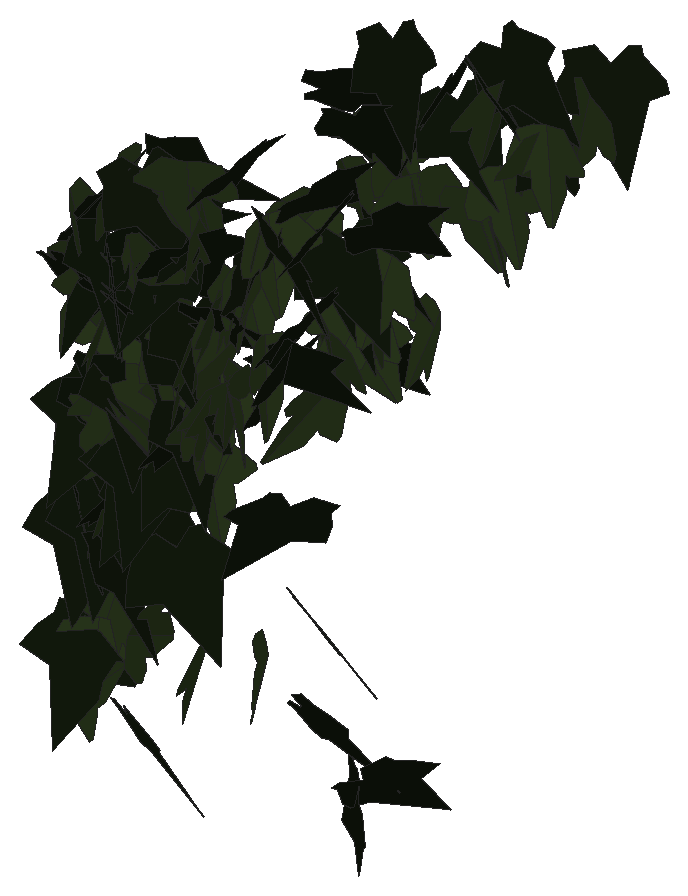
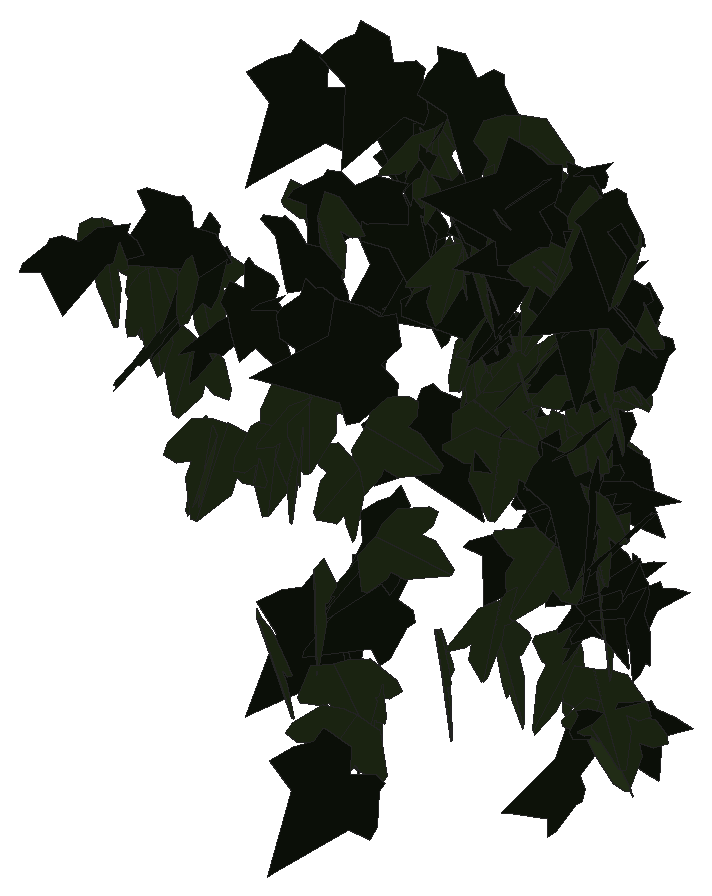
# SketchUp Ruby script. Lengths in inches.
U = 1.inch
M = Sketchup.active_model
def pt(a) = Geom::Point3d.new(a.map { |v| v * U })
def face(e, loops, mat)
  f = e.add_face(loops[0].map { |a| pt(a) })
  loops[1..].each { |l| e.add_face(l.map { |a| pt(a) }).erase! }
  f.material = f.back_material = mat if mat
  f
end
# faces: each face lists its corners as indices into pts; further lists are holes
def faces(e, pts, list, mat = nil) = list.each { |f| face(e, (f[0].is_a?(Array) ? f : [f]).map { |l| l.map { |i| pts[i] } }, mat) }
# xy, xz, yz: faces in a plane at the given z, y or x. An outline is a flat list of corners, or four numbers for a rectangle; further outlines are holes
def ring(l) = l.size == 4 ? [[l[0], l[1]], [l[2], l[1]], [l[2], l[3]], [l[0], l[3]]] : l.each_slice(2).to_a
def flat(e, list, mat, &to3) = list.each { |f| face(e, (f[0].is_a?(Array) ? f : [f]).map { |l| ring(l).map { |u, v| to3.(u, v) } }, mat) }
def xy(e, z, list, mat = nil) = flat(e, list, mat) { |x, y| [x, y, z] }
def xz(e, y, list, mat = nil) = flat(e, list, mat) { |x, z| [x, y, z] }
def yz(e, x, list, mat = nil) = flat(e, list, mat) { |y, z| [x, y, z] }
def lines(e, pts, list) = list.each { |a, b| e.add_line(pt(pts[a]), pt(pts[b])) }
# prism: a flat outline (further loops are holes) pulled along v
def prism(e, loops, v, mat = nil)
  f = face(e, loops, mat); d = Geom::Vector3d.new(v.map { |x| x * U })
  f.pushpull(f.normal.samedirection?(d) ? d.length : -d.length)
end
def box(e, o, s, mat = nil) = prism(e, [[o, [o[0] + s[0], o[1], o[2]], [o[0] + s[0], o[1] + s[1], o[2]], [o[0], o[1] + s[1], o[2]]]], [0, 0, s[2]], mat)
def at(x, y, z, deg = 0) = Geom::Transformation.translation(pt([x, y, z])) * Geom::Transformation.rotation(ORIGIN, Z_AXIS, deg.degrees)
def axes(o, x, y, z) = Geom::Transformation.new([*x, 0, *y, 0, *z, 0, *pt(o).to_a, 1])
def part(name) = M.definitions.add(name)
# library, detail: a bought-in or finely detailed component or shape, given as its bounding box
def library(name, o, s) = part(name).tap { |d| box(d.entities, o, s) }
def detail(e, o, s) = box(e.add_group.entities, o, s)
def put(e, d, t, mat = nil) = e.add_instance(d, t).tap { |i| i.material = mat if mat }
def group(e, t, mat = nil) = e.add_group.tap { |g| g.transformation = t; g.material = mat if mat }.entities
root = M.entities
M.materials.add("efeu1").color = [18, 25, 13]
M.materials.add("efeu2").color = [43, 57, 29]
c1 = part("ivyleaf_9")
p = [[1.54,2.16,1.25],[1.36,2.04,1.19],[-0.21,0.99,0.68],[-0.71,1.11,0.82],[-0.85,0.86,0.67],[-0.8,0.17,0.21],
  [-0.9,-0.01,0.1],[-0.67,-0.16,-0.02],[-0.08,-0.08,-0.05],[-0.03,-0.6,-0.4],[0.65,-0.88,-0.66],[0.83,-0.6,-0.49],
  [1.29,-0.42,-0.43],[1.8125,-0.07,-0.26],[1.21,0.44,0.15]]
faces(c1.entities,p,[[0,1,2,3,4,5,6,7,8,9,10,11,12,13,14]],"efeu1")
c2 = part("ivyleaf_10")
p = [[0,0.5,-0.03],[-0.0625,2.02,-0.43],[-0.19,2.01,-0.46],[-0.54,1.05,-0.29],[-0.52,0.625,-0.18],[-0.83,0.76,-0.28],
  [-1.16,0.64,-0.33],[-1.15,0.33,-0.24],[-0.77,-0.39,0.02],[-0.3,-0.51,0.16],[0.04,-0.48,0.23],[-0.02,2.01,-0.4375],
  [-0.06,2.01,-0.43],[0.04,-0.49,0.23],[0.67,-0.49,0.14],[1.38,0.36,-0.2],[1.375,0.51,-0.24],[0.81,0.65,-0.19],
  [0.62,0.59,-0.15],[0.6,1.09,-0.28],[0.5,1.23,-0.31]]
faces(c2.entities,p,[[0,1,2,3,4,5,6,7,8,9,10],[11,12,0,13,14,15,16,17,18,19,20]],"efeu2")
put(root,c1,axes([47.6,222.98,241.15],[0.28604,-0.36805,0.18089],[0.10443,-0.14791,-0.46607],[0.39658,0.30441,-0.00775]))
put(root,c2,axes([47.37,222.98,241.04],[-0.14695,0.39138,-0.27427],[-0.05131,-0.2982,-0.39805],[-0.47515,-0.08884,0.12781]))
put(root,c1,axes([45.58,223.13,237.33],[-0.35883,-0.34791,-0.01403],[0.06783,-0.05009,-0.49284],[0.34152,-0.3556,0.08314]))
put(root,c1,axes([45.51,223.15,237.27],[-0.12119,-0.47664,0.09015],[-0.0015,-0.09255,-0.49136],[0.48509,-0.11937,0.021]))
put(root,c1,axes([45.03,222.95,235.92],[0.29145,-0.40527,0.02852],[0.01419,-0.02492,-0.49918],[0.40602,0.29178,-0.00302]))
put(root,c1,axes([44.71,223.06,234.62],[-0.35713,-0.33851,-0.08871],[0.0584,0.06733,-0.49199],[0.34503,-0.36177,-0.00856]))
put(root,c2,axes([45.1875,222.87,237.78],[-0.41971,-0.04897,0.26729],[-0.25366,-0.10581,-0.41769],[0.09747,-0.48622,0.06398]))
put(root,c2,axes([46.34,222.83,241.66],[-0.44608,-0.22491,0.02083],[-0.01528,-0.01595,-0.49951],[0.22535,-0.44628,0.00736]))
put(root,c1,axes([44.92,223.09,240.11],[0.07095,-0.49203,0.05358],[0.00626,-0.05323,-0.49712],[0.4949,0.07121,-0.0014]))
put(root,c1,axes([44.87,223.05,240.09],[-0.42662,-0.06259,-0.25313],[0.25792,-0.02984,-0.4273],[0.03838,-0.49517,0.05775]))
put(root,c2,axes([47.5,222.91,239.53],[-0.0551,0.4761,-0.14244],[-0.00281,-0.14361,-0.47892],[-0.49695,-0.05198,0.0185]))
put(root,c2,axes([44.7,223.02,233.87],[0.14859,-0.36574,-0.30685],[0.26499,-0.20414,0.37163],[-0.39712,-0.27306,0.13317]))
put(root,c1,axes([46.1,222.92,236.33],[-0.11764,-0.34267,-0.34459],[0.22985,0.27315,-0.35009],[0.42817,-0.24077,0.09326]))
put(root,c2,axes([46.55,223.02,239.73],[0.24723,-0.41637,0.12454],[0.07019,-0.10314,-0.48418],[0.42889,0.25689,0.00745]))
put(root,c2,axes([44.64,222.82,240.6],[-0.20643,0.45476,-0.02403],[-0.00018,-0.02646,-0.4993],[-0.4554,-0.20613,0.01108]))
put(root,c2,axes([45.82,222.85,240.27],[-0.46736,0.00036,0.1777],[-0.17738,-0.03109,-0.46644],[0.01072,-0.49903,0.02919]))
put(root,c1,axes([47.76,222.95,237.49],[-0.01009,0.32824,-0.37704],[-0.10454,-0.37016,-0.31946],[-0.48885,0.07239,0.0761]))
put(root,c1,axes([45.58,222.93,241.36],[0.08904,-0.4323,-0.23493],[0.06047,0.24655,-0.43076],[0.48828,0.04829,0.09619]))
put(root,c1,axes([45.23,222.63,241.15],[-0.06272,0.47356,0.14768],[-0.06747,0.13933,-0.47543],[-0.49144,-0.07957,0.04643]))
put(root,c1,axes([44.9,223.15,239.875],[0.03196,-0.00013,-0.49898],[0.47505,-0.15296,0.03047],[-0.15266,-0.47603,-0.00966]))
put(root,c2,axes([46.62,223.02,238.57],[0.13599,-0.47813,0.05381],[0.01,-0.0531,-0.49707],[0.48105,0.13627,-0.00488]))
put(root,c2,axes([46.13,223.06,239.05],[0.2724,-0.40437,0.11081],[0.07632,-0.08211,-0.48727],[0.41228,0.28238,0.01699]))
put(root,c2,axes([46.47,223.03,238.36],[0.03089,-0.49446,0.0675],[0.00051,-0.06759,-0.49541],[0.49904,0.03067,-0.00368]))
put(root,c1,axes([45.93,223.17,240.29],[-0.45951,-0.0891,-0.17581],[0.1917,-0.09836,-0.4512],[0.04582,-0.48207,0.12455]))
put(root,c2,axes([46.26,222.93,241.26],[-0.41596,-0.09564,0.26044],[-0.25167,-0.06753,-0.42674],[0.1168,-0.4861,0.00804]))
put(root,c2,axes([44.64,223.17,239.54],[-0.00824,-0.42593,0.26176],[0.03234,-0.2617,-0.42481],[0.49888,0.00993,0.03186]))
put(root,c2,axes([45.09,222.99,238.12],[-0.0935,0.04522,-0.48909],[0.46125,-0.16305,-0.10325],[-0.16883,-0.4705,-0.01123]))
put(root,c1,axes([47.1,222.65,242.05],[0.00869,0.49275,0.08441],[-0.03311,0.0848,-0.49164],[-0.49883,0.00295,0.0341]))
put(root,c2,axes([47.56,222.9,241.22],[0.10794,0.48798,-0.01486],[0.00353,-0.01599,-0.49973],[-0.4882,0.10778,-0.00689]))
put(root,c2,axes([44.77,222.91,239.87],[-0.49251,-0.02626,0.08211],[-0.08067,-0.02749,-0.49268],[0.03039,-0.49855,0.02284]))
put(root,c1,axes([46.09,223.15,238.11],[0.11345,-0.48539,0.0391],[0.01037,-0.03773,-0.49847],[0.48685,0.11391,0.0015]))
put(root,c1,axes([48.16,222.86,234.87],[0.48306,-0.09603,0.08621],[0.08554,-0.0118,-0.49249],[0.09662,0.49055,0.00503]))
put(root,c1,axes([48.375,222.78,241.625],[-0.16599,0.4716,0.00615],[0.00009,0.00655,-0.49996],[-0.47164,-0.16597,-0.00226]))
put(root,c2,axes([44.9,222.98,239.15],[0.21957,-0.44175,-0.08151],[-0.04878,0.06675,-0.49312],[0.44656,0.2245,-0.01379]))
put(root,c1,axes([47.67,222.55,239.13],[0.09531,0.21275,0.44233],[0.10934,0.43006,-0.23041],[-0.4785,0.14065,0.03545]))
put(root,c2,axes([46.34,223.05,234.98],[0.20444,-0.45618,0.0102],[0.00335,-0.00967,-0.4999],[0.45628,0.20447,-0.0009]))
put(root,c1,axes([47.47,222.68,240.75],[-0.13862,0.38287,0.29017],[-0.12009,0.2648,-0.40677],[-0.46515,-0.18247,0.01855]))
put(root,c1,axes([44.87,222.89,239.39],[0.46589,-0.1151,0.14037],[0.13818,-0.02586,-0.47983],[0.11771,0.48588,0.00772]))
put(root,c1,axes([44.74,223.25,236.36],[-0.05848,-0.49573,0.02878],[-0.0111,-0.02767,-0.49911],[0.49644,-0.05902,-0.00777]))
put(root,c1,axes([44.375,222.84,239.73],[0.49918,-0.02713,0.00929],[0.01052,0.02252,-0.49938],[0.02668,0.49876,0.02305]))
put(root,c1,axes([44.5,223.24,236.21],[-0.14334,-0.47866,-0.01836],[0.02143,0.01274,-0.49938],[0.47853,-0.14395,0.01687]))
put(root,c1,axes([48.03,222.84,240.19],[-0.12703,0.48156,-0.04433],[-0.00004,-0.04584,-0.49789],[-0.48359,-0.12649,0.01168]))
put(root,c2,axes([46.77,222.99,238.75],[-0.08312,-0.48753,-0.07349],[-0.0059,0.0755,-0.49423],[0.49301,-0.0813,-0.01831]))
put(root,c2,axes([47.1,223.01,240.28],[0.31561,-0.3772,-0.09003],[-0.0171,0.10244,-0.4891],[0.38742,0.31181,0.05176]))
put(root,c1,axes([44.18,223.2,236.24],[0.06907,-0.03833,-0.49372],[0.49411,-0.02782,0.07128],[-0.03293,-0.49775,0.03404]))
put(root,c2,axes([44.71,223.04,234.6],[0.46843,0.17468,-0.00779],[-0.01618,0.02112,-0.49929],[-0.17411,0.46802,0.02544]))
put(root,c1,axes([44.68,223.31,237.74],[-0.39387,-0.30628,-0.03253],[0.06808,-0.03508,-0.4941],[0.30038,-0.39365,0.06933]))
put(root,c1,axes([46.29,222.79,240.62],[0.21685,0.44719,-0.05476],[-0.0266,-0.04796,-0.49698],[-0.44975,0.21845,0.00299]))
put(root,c1,axes([46.1,223.1875,239.46],[0.09539,-0.48653,-0.06474],[-0.02045,0.06195,-0.49573],[0.49039,0.09722,-0.00808]))
put(root,c1,axes([45.26,223.08,233.65],[0.39625,-0.2893,0.09641],[0.07937,-0.05479,-0.49061],[0.29443,0.40411,0.0025]))
put(root,c1,axes([44.68,222.9375,238.1875],[0.10643,0.0448,-0.48648],[0.3771,0.30901,0.11095],[0.3106,-0.39052,0.03198]))
put(root,c2,axes([46.37,223.04,238.22],[-0.02295,0.49511,-0.06587],[0.00068,-0.0659,-0.49564],[-0.49947,-0.02284,0.00236]))
put(root,c1,axes([45.78,223.13,239.02],[0.2673,-0.41985,-0.04773],[0.02298,0.07084,-0.49442],[0.42192,0.26213,0.05717]))
put(root,c2,axes([46.86,223,238.78],[-0.2812,0.41185,0.03617],[-0.04683,0.01174,-0.49766],[-0.41078,-0.28327,0.03197]))
put(root,c1,axes([45.08,223.35,238.19],[-0.00409,-0.49753,0.04951],[0.02716,-0.04966,-0.49679],[0.49924,-0.00138,0.02744]))
put(root,c1,axes([48.86,222.92,233.83],[0.06026,0.00487,-0.49633],[-0.49069,0.07588,-0.05883],[0.07475,0.49418,0.01393]))
put(root,c1,axes([46.3,223.01,240.76],[-0.30761,0.34901,0.18321],[-0.17243,0.08983,-0.46065],[-0.35446,-0.34658,0.06509]))
put(root,c1,axes([47.67,222.88,239.56],[0.4556,0.17899,0.10192],[0.09566,0.03525,-0.4895],[-0.18242,0.46553,-0.00212]))
put(root,c2,axes([45.83,223.12,239.05],[0.11955,0.48421,-0.03528],[-0.00429,-0.03528,-0.49874],[-0.48548,0.11955,-0.00429]))
put(root,c2,axes([45.01,223.21,238.09],[-0.16768,-0.46946,0.03862],[0.00628,-0.04322,-0.49809],[0.471,-0.16656,0.02039]))
put(root,c2,axes([46.43,222.95,240.97],[0.12144,-0.37164,-0.31167],[0.02268,0.32529,-0.37904],[0.4845,0.07792,0.09586]))
put(root,c2,axes([45.32,223.1,238.17],[0.46774,-0.13659,-0.11208],[-0.06879,0.15137,-0.47155],[0.16275,0.45654,0.12281]))
put(root,c2,axes([46.64,223.2,239.9375],[0.36195,-0.33847,-0.06659],[-0.04212,0.05244,-0.49546],[0.34238,0.36427,0.00945]))
put(root,c1,axes([44.95,223.01,237.82],[0.47502,-0.05907,-0.14444],[-0.13818,0.05582,-0.47727],[0.07251,0.49335,0.03671]))
put(root,c2,axes([44.83,223.14,235.01],[0.48673,0.00901,-0.11409],[-0.11352,0.10122,-0.47631],[0.01451,0.48957,0.10058]))
put(root,c2,axes([45.16,222.89,241.07],[-0.01738,-0.29817,-0.40099],[0.05405,0.39776,-0.2981],[0.49677,-0.05371,0.01841]))
put(root,c1,axes([46.4,223.05,239.54],[0.39537,-0.09885,0.28968],[0.30132,0.04257,-0.39673],[0.05377,0.48828,0.09323]))
put(root,c2,axes([46.6,222.8,239.16],[0.05121,-0.00824,-0.4973],[0.03642,0.49865,-0.00451],[0.49604,-0.03576,0.05167]))
put(root,c1,axes([46.14,223.07,238],[-0.10601,0.47487,-0.11514],[0.00085,-0.11765,-0.48596],[-0.48863,-0.10323,0.02414]))
put(root,c1,axes([49.05,222.89,234.24],[0.36148,0.31717,0.13687],[0.09307,0.10136,-0.48069],[-0.33267,0.373,0.01424]))
put(root,c2,axes([44.9375,223.28,239.01],[0.42806,0.25282,-0.0533],[-0.04139,-0.0347,-0.49707],[-0.25504,0.42997,-0.00878]))
put(root,c2,axes([45.55,222.88,234.98],[0.05489,0.21099,0.44997],[-0.20513,0.42196,-0.17284],[-0.45267,-0.16563,0.13288]))
put(root,c1,axes([45.09,223.2,236.75],[-0.15317,0.44386,-0.17185],[0.01282,-0.17661,-0.46759],[-0.47579,-0.14765,0.04272]))
put(root,c1,axes([45.34,222.96,239.89],[-0.05653,0.47457,0.14694],[-0.02829,0.14458,-0.4778],[-0.49599,-0.06233,0.0105]))
put(root,c2,axes([44.72,223.25,236.35],[0.22364,-0.43838,-0.08837],[0.0018,0.09968,-0.48996],[0.44719,0.21883,0.04616]))
put(root,c1,axes([48.16,222.91,242.01],[0.1857,0.43951,0.14949],[0.01386,0.15569,-0.47494],[-0.46403,0.18054,0.04564]))
put(root,c1,axes([45.43,222.92,240.63],[0.04624,0.2487,-0.43129],[0.06207,0.42689,0.25281],[0.49397,-0.07692,0.00861]))
put(root,c1,axes([47.84,223.19,236.02],[0.47244,-0.12893,-0.10089],[-0.09196,0.04594,-0.48932],[0.13545,0.4809,0.0197]))
put(root,c1,axes([45.19,223.21,236.84],[0.30996,-0.31677,-0.23147],[-0.01529,0.28501,-0.41053],[0.39203,0.26158,0.167]))
put(root,c1,axes([44.68,222.94,240.42],[0.26203,0.27524,0.32494],[0.20368,0.25405,-0.37944],[-0.37397,0.33122,0.02102]))
put(root,c1,axes([44.3,223.625,237.25],[0.10252,-0.48888,0.02205],[0.04527,-0.01296,-0.49778],[0.48728,0.10406,0.0416]))
put(root,c2,axes([46.83,223.34,240.13],[0.05477,0.49243,0.06716],[-0.00225,0.06781,-0.49537],[-0.49699,0.05396,0.00965]))
put(root,c2,axes([44.74,223.46,237.62],[0.45912,-0.18434,-0.07229],[-0.04157,0.08874,-0.4903],[0.1936,0.45623,0.06616]))
put(root,c2,axes([46.15,223.61,238.46],[0.28174,0.27194,-0.31092],[-0.25306,-0.18383,-0.39009],[-0.32647,0.37717,0.03406]))
put(root,c2,axes([45.4375,223.16,240.33],[0.12766,0.35677,0.32621],[-0.09178,0.34915,-0.34594],[-0.47464,0.02845,0.15463]))
put(root,c2,axes([46.97,223.43,234.86],[0.25969,-0.37001,-0.21367],[-0.08726,0.19883,-0.45039],[0.41827,0.27121,0.03869]))
put(root,c1,axes([45.59,223.45,241.23],[0.32913,-0.05039,0.37301],[0.36763,-0.06325,-0.33293],[0.08074,0.49342,-0.00459]))
put(root,c1,axes([44.72,223.34,237.78],[0.04145,0.01105,-0.49816],[-0.44303,0.22959,-0.03178],[0.22804,0.44404,0.02882]))
put(root,c1,axes([48.84,223.3125,241.63],[0.33144,0.35479,0.11948],[0.07649,0.09203,-0.48547],[-0.36647,0.34008,0.00673]))
put(root,c2,axes([45.89,223.7,238.02],[0.44745,0.20079,0.09732],[0.07341,0.07346,-0.48909],[-0.21071,0.45198,0.03626]))
put(root,c1,axes([47.99,223.8125,240.84],[-0.11655,-0.33753,-0.34999],[0.13584,0.32296,-0.35671],[0.46686,-0.17824,0.01642]))
put(root,c1,axes([44.91,223.55,237.91],[-0.04542,0.47484,0.14988],[-0.01888,0.14875,-0.47699],[-0.49757,-0.04899,0.00442]))
put(root,c2,axes([48.43,223.94,240.54],[0.49414,-0.05231,-0.05557],[-0.05515,0.00688,-0.4969],[0.05275,0.49721,0.00103]))
put(root,c2,axes([47.14,224.4,238.13],[0.01704,0.35442,-0.35227],[-0.26805,-0.29099,-0.30573],[-0.42173,0.19927,0.18009]))
put(root,c2,axes([44.85,224.13,237.16],[0.41742,0.10559,0.25419],[0.21606,0.16037,-0.42142],[-0.17053,0.46166,0.08825]))
put(root,c2,axes([45.27,224.59,236.48],[0.03412,0.49871,-0.01096],[0.00177,-0.01111,-0.49987],[-0.49883,0.03408,-0.00252]))
put(root,c1,axes([46.51,226.14,239.43],[0.40457,-0.20822,-0.20729],[-0.17005,0.12172,-0.45417],[0.2396,0.43798,0.02767]))
put(root,c1,axes([46.46,226.61,241.84],[-0.23572,-0.16731,-0.40798],[0.39898,0.11605,-0.27811],[0.18775,-0.45666,0.0788]))
put(root,c1,axes([46.15,226.32,240.85],[0.37287,0.31422,-0.11063],[-0.09093,-0.06374,-0.48751],[-0.32047,0.38367,0.00961]))
put(root,c1,axes([45.28,226.96,238.27],[0.24144,-0.43771,0.01067],[0.01072,-0.00627,-0.49985],[0.43771,0.2416,0.00635]))
put(root,c2,axes([44.82,227.1,238.7],[0.17868,0.27488,-0.37751],[-0.24396,-0.28971,-0.32642],[-0.39819,0.30085,0.03059]))
put(root,c2,axes([48.48,226.99,240.98],[0.48619,-0.03265,0.11202],[0.11548,0.06584,-0.48201],[0.01673,0.49457,0.07157]))
put(root,c1,axes([45.29,226.78,240.75],[0.38268,0.00603,0.32175],[0.30868,0.13443,-0.36965],[-0.09097,0.48155,0.09916]))
put(root,c1,axes([46.9375,227.11,241.27],[-0.27916,0.30401,-0.28222],[0.1864,-0.21197,-0.4127],[-0.37057,-0.33563,0.00501]))
put(root,c2,axes([47.78,227.03,240.15],[0.46675,-0.00076,0.1793],[0.17706,0.08076,-0.46057],[-0.02826,0.49343,0.07565]))
put(root,c2,axes([47.6,227.15,241.28],[-0.00445,-0.49854,0.03793],[0.01452,-0.03805,-0.49834],[0.49977,-0.00334,0.01482]))
put(root,c2,axes([45.39,227.2,239.38],[-0.35938,0.19162,-0.29005],[0.2294,-0.18272,-0.40495],[-0.26119,-0.42414,0.04342]))
put(root,c2,axes([48.27,227.19,240.86],[-0.04101,-0.49796,-0.01873],[0.01204,0.0178,-0.49954],[0.49817,-0.04142,0.01053]))
put(root,c1,axes([47.55,227,241.51],[0.4403,-0.09077,-0.21885],[-0.20503,0.08546,-0.44795],[0.11872,0.48421,0.03803]))
put(root,c1,axes([46.99,227.22,240.92],[0.09416,-0.45062,-0.19514],[0.03861,0.20487,-0.45446],[0.48953,0.07052,0.07338]))
put(root,c2,axes([46.4,227.1875,239.59],[-0.22564,-0.4423,-0.05883],[0.1103,0.00859,-0.48761],[0.43234,-0.23302,0.0937]))
put(root,c2,axes([45.95,227.19,240.38],[-0.34671,-0.36025,0.0028],[-0.00155,-0.00239,-0.49999],[0.36026,-0.34671,0.00054]))
put(root,c1,axes([47.7,227.21,241.9],[-0.03863,-0.10368,-0.48761],[0.39449,0.29264,-0.09348],[0.30477,-0.39193,0.05919]))
put(root,c2,axes([46.05,227.16,240],[0.01891,0.49872,0.03038],[-0.00119,0.03044,-0.49907],[-0.49964,0.0188,0.00234]))
put(root,c2,axes([45.73,227.28,237.8],[0.22178,-0.44658,-0.03715],[0.07721,0.07891,-0.48766],[0.44142,0.21057,0.10396]))
put(root,c2,axes([46.08,227.28,239.66],[-0.37433,0.32597,0.06017],[-0.09514,-0.01872,-0.49051],[-0.31753,-0.37867,0.07605]))
put(root,c2,axes([44.99,227.34,236.84],[-0.44657,0.20391,0.09482],[-0.09365,0.02303,-0.49061],[-0.20445,-0.45595,0.01762]))
put(root,c2,axes([48.86,227.42,241.42],[-0.42755,0.1691,0.19648],[-0.21776,-0.02869,-0.44917],[-0.14064,-0.46966,0.09818]))
put(root,c2,axes([46.99,227.56,239.4375],[-0.47091,-0.13695,-0.09739],[0.10346,-0.00792,-0.48912],[0.13243,-0.48081,0.0358]))
put(root,c1,axes([47.8125,228,240.4375],[-0.11585,-0.32024,0.3661],[0.04272,-0.38158,-0.32026],[0.48451,-0.04292,0.11578]))
put(root,c2,axes([45.01,227.7,237.07],[0.44189,0.172,-0.15859],[-0.16314,-0.01642,-0.47235],[-0.1677,0.4692,0.04161]))
put(root,c2,axes([47.07,227.69,239.38],[-0.32147,0.36904,-0.1023],[0.06485,-0.07917,-0.48941],[-0.37743,-0.32793,0.00304]))
put(root,c2,axes([46.07,227.79,237.3],[0.36017,-0.33181,-0.1009],[-0.08303,0.05874,-0.48955],[0.33672,0.3694,-0.01279]))
put(root,c1,axes([48.7,228.01,241.6875],[-0.1075,-0.43912,-0.21358],[0.05087,0.20743,-0.45209],[0.48565,-0.11893,0.00008]))
put(root,c2,axes([44.72,228.07,236.62],[-0.39705,-0.19324,-0.23454],[0.25187,0.00666,-0.43188],[0.17003,-0.4611,0.09205]))
put(root,c1,axes([44.5,228.31,236.2],[0.41007,0.282,0.04815],[0.02571,0.04748,-0.49708],[-0.28492,0.41015,0.02444]))
